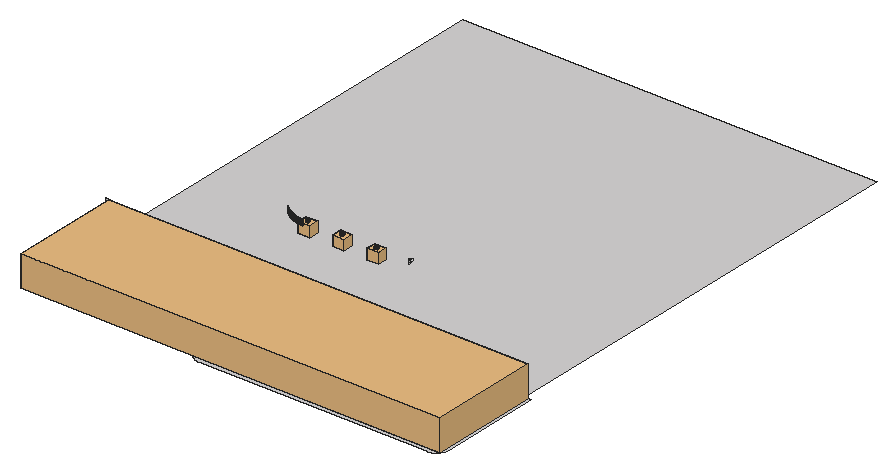
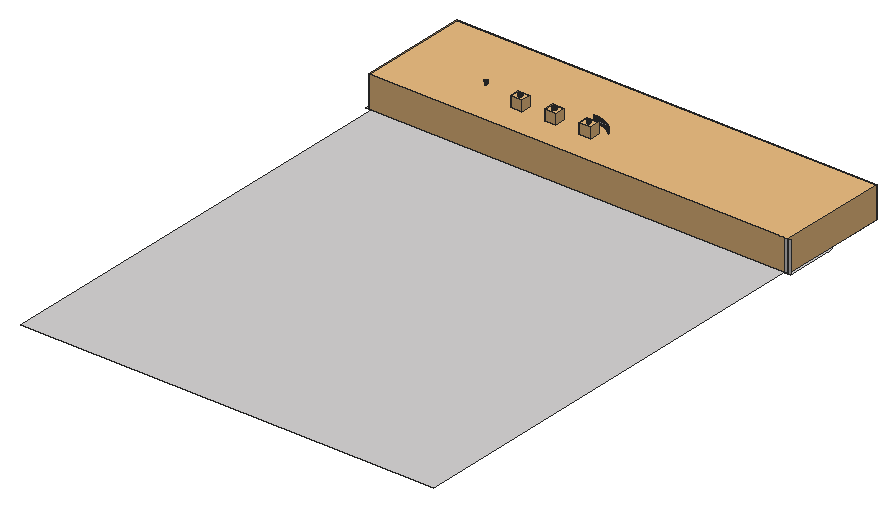
# SketchUp Ruby script. Lengths in inches.
U = 1.inch
M = Sketchup.active_model
def pt(a) = Geom::Point3d.new(a.map { |v| v * U })
def face(e, loops, mat)
  f = e.add_face(loops[0].map { |a| pt(a) })
  loops[1..].each { |l| e.add_face(l.map { |a| pt(a) }).erase! }
  f.material = f.back_material = mat if mat
  f
end
# faces: each face lists its corners as indices into pts; further lists are holes
def faces(e, pts, list, mat = nil) = list.each { |f| face(e, (f[0].is_a?(Array) ? f : [f]).map { |l| l.map { |i| pts[i] } }, mat) }
# xy, xz, yz: faces in a plane at the given z, y or x. An outline is a flat list of corners, or four numbers for a rectangle; further outlines are holes
def ring(l) = l.size == 4 ? [[l[0], l[1]], [l[2], l[1]], [l[2], l[3]], [l[0], l[3]]] : l.each_slice(2).to_a
def flat(e, list, mat, &to3) = list.each { |f| face(e, (f[0].is_a?(Array) ? f : [f]).map { |l| ring(l).map { |u, v| to3.(u, v) } }, mat) }
def xy(e, z, list, mat = nil) = flat(e, list, mat) { |x, y| [x, y, z] }
def xz(e, y, list, mat = nil) = flat(e, list, mat) { |x, z| [x, y, z] }
def yz(e, x, list, mat = nil) = flat(e, list, mat) { |y, z| [x, y, z] }
def lines(e, pts, list) = list.each { |a, b| e.add_line(pt(pts[a]), pt(pts[b])) }
# prism: a flat outline (further loops are holes) pulled along v
def prism(e, loops, v, mat = nil)
  f = face(e, loops, mat); d = Geom::Vector3d.new(v.map { |x| x * U })
  f.pushpull(f.normal.samedirection?(d) ? d.length : -d.length)
end
def box(e, o, s, mat = nil) = prism(e, [[o, [o[0] + s[0], o[1], o[2]], [o[0] + s[0], o[1] + s[1], o[2]], [o[0], o[1] + s[1], o[2]]]], [0, 0, s[2]], mat)
def at(x, y, z, deg = 0) = Geom::Transformation.translation(pt([x, y, z])) * Geom::Transformation.rotation(ORIGIN, Z_AXIS, deg.degrees)
def axes(o, x, y, z) = Geom::Transformation.new([*x, 0, *y, 0, *z, 0, *pt(o).to_a, 1])
def part(name) = M.definitions.add(name)
# library, detail: a bought-in or finely detailed component or shape, given as its bounding box
def library(name, o, s) = part(name).tap { |d| box(d.entities, o, s) }
def detail(e, o, s) = box(e.add_group.entities, o, s)
def put(e, d, t, mat = nil) = e.add_instance(d, t).tap { |i| i.material = mat if mat }
def group(e, t, mat = nil) = e.add_group.tap { |g| g.transformation = t; g.material = mat if mat }.entities
root = M.entities
M.materials.add("T METAL").color = [42, 41, 39]
M.materials.add("[Quartz Light Brown]").color = [215, 212, 212]
c1 = library("3",[-5.26,-4.28,-11.86],[13.52,11.56,11.86])
c2 = library("Group\#48",[0,0,0],[483,127.5,40])
xy(root,396,[[215.8,143,480.2,143,480.39,143.01,480.59,143.01,480.79,143.02,480.98,143.03,481.18,143.05,481.37,143.0625,481.57,143.08,481.76,143.1,481.96,143.13,482.15,143.16,482.35,143.18,482.54,143.22,482.73,143.25,482.93,143.29,483.5,143.41,483.88,143.51,484.07,143.5625,484.26,143.62,484.45,143.67,484.64,143.73,484.82,143.8,485.01,143.86,485.19,143.93,485.56,144.07,485.74,144.14,486.46,144.46,486.63,144.55,486.81,144.63,486.98,144.73,487.16,144.82,487.33,144.91,487.84,145.21,488,145.3125,488.17,145.42,488.33,145.53,488.5,145.64,488.82,145.86,488.97,145.98,489.29,146.22,489.44,146.34,489.59,146.47,489.74,146.59,490.04,146.85,490.18,146.99,490.33,147.12,490.47,147.26,490.61,147.39,490.74,147.53,490.88,147.67,491.01,147.82,491.15,147.96,491.41,148.26,491.53,148.41,491.66,148.56,491.78,148.71,492.02,149.03,492.14,149.18,492.36,149.5,492.47,149.67,492.58,149.83,492.6875,150,492.79,150.16,493.09,150.67,493.18,150.84,493.27,151.02,493.37,151.19,493.45,151.37,493.54,151.54,493.86,152.26,493.93,152.44,494.07,152.81,494.14,152.99,494.2,153.18,494.27,153.36,494.33,153.55,494.38,153.74,494.4375,153.93,494.49,154.12,494.59,154.5,494.71,155.07,494.75,155.27,494.78,155.46,494.82,155.65,494.84,155.85,494.87,156.04,494.9,156.24,494.92,156.43,494.9375,156.63,494.95,156.82,494.97,157.02,494.98,157.21,494.99,157.41,494.99,157.61,495,157.8,495,276.5,488,276.5,488,787,7,787,7,276.5,0,276.5,0,222.76,0.01,222.53,0.01,222.29,0.02,222.06,0.04,221.82,0.06,221.59,0.08,221.35,0.1,221.12,0.125,220.88,0.15,220.65,0.1875,220.42,0.22,220.18,0.3,219.72,0.35,219.49,0.39,219.26,0.44,219.03,0.5,218.8,0.55,218.57,0.61,218.34,0.68,218.11,0.74,217.89,0.81,217.66,0.88,217.4375,0.96,217.21,1.03,216.99,1.11,216.77,1.2,216.55,1.28,216.33,1.46,215.89,1.56,215.68,1.65,215.46,1.75,215.25,1.86,215.04,1.96,214.83,2.18,214.41,2.3,214.2,2.41,214,2.65,213.6,2.78,213.39,2.9,213.2,3.03,213,3.17,212.8,3.3,212.61,3.4375,212.42,3.58,212.23,3.72,212.04,3.86,211.86,4.01,211.67,4.16,211.49,4.3125,211.31,4.47,211.13,4.625,210.96,4.78,210.78,4.94,210.61,5.11,210.44,5.27,210.27,5.44,210.11,5.61,209.94,5.78,209.78,5.96,209.625,6.13,209.47,6.31,209.3125,6.49,209.16,6.67,209.01,6.86,208.86,7.04,208.72,7.23,208.58,7.42,208.4375,7.61,208.3,7.8,208.17,8,208.03,8.2,207.9,8.39,207.78,8.6,207.65,9,207.41,9.2,207.3,9.41,207.18,9.83,206.96,10.04,206.86,10.25,206.75,10.46,206.65,10.68,206.56,10.89,206.46,11.33,206.28,11.55,206.2,11.77,206.11,11.99,206.03,12.21,205.96,12.4375,205.88,12.66,205.81,12.89,205.74,13.11,205.68,13.34,205.61,13.57,205.55,13.8,205.5,14.03,205.44,14.26,205.39,14.49,205.35,14.72,205.3,15.18,205.22,15.42,205.1875,15.65,205.15,15.88,205.125,16.12,205.1,16.35,205.08,16.59,205.06,16.82,205.04,17.06,205.02,17.29,205.01,17.53,205.01,17.76,205,201,205,201,157.8,201.01,157.61,201.01,157.41,201.02,157.21,201.03,157.02,201.05,156.82,201.0625,156.63,201.08,156.43,201.1,156.24,201.13,156.04,201.16,155.85,201.18,155.65,201.22,155.46,201.25,155.27,201.29,155.07,201.41,154.5,201.51,154.12,201.5625,153.93,201.62,153.74,201.67,153.55,201.73,153.36,201.8,153.18,201.86,152.99,201.93,152.81,202.07,152.44,202.14,152.26,202.46,151.54,202.55,151.37,202.63,151.19,202.73,151.02,202.82,150.84,202.91,150.67,203.21,150.16,203.3125,150,203.42,149.83,203.53,149.67,203.64,149.5,203.86,149.18,203.98,149.03,204.22,148.71,204.34,148.56,204.47,148.41,204.59,148.26,204.85,147.96,204.99,147.82,205.12,147.67,205.26,147.53,205.39,147.39,205.53,147.26,205.67,147.12,205.82,146.99,205.96,146.85,206.26,146.59,206.41,146.47,206.56,146.34,206.71,146.22,207.03,145.98,207.18,145.86,207.5,145.64,207.67,145.53,207.83,145.42,208,145.3125,208.16,145.21,208.67,144.91,208.84,144.82,209.02,144.73,209.19,144.63,209.37,144.55,209.54,144.46,210.26,144.14,210.44,144.07,210.81,143.93,210.99,143.86,211.18,143.8,211.36,143.73,211.55,143.67,211.74,143.62,211.93,143.5625,212.12,143.51,212.5,143.41,213.07,143.29,213.27,143.25,213.46,143.22,213.65,143.18,213.85,143.16,214.04,143.13,214.24,143.1,214.43,143.08,214.63,143.0625,214.82,143.05,215.02,143.03,215.21,143.02,215.41,143.01,215.61,143.01]],"[Quartz Light Brown]")
xy(root,483,[[224.9375,287.7,224.78,287.71,224.47,287.77,224.32,287.82,224.18,287.88,224.04,287.95,223.9,288.03,223.77,288.12,223.65,288.22,223.54,288.33,223.44,288.45,223.26,288.71,223.19,288.85,223.13,288.99,223.08,289.14,223.04,289.29,223,289.61,223,289.76,223.01,289.92,223.04,290.08,223.07,290.23,223.12,290.38,223.18,290.52,223.25,290.66,223.33,290.8,223.42,290.93,223.52,291.05,223.63,291.16,223.75,291.26,223.875,291.35,224.01,291.4375,224.15,291.51,224.29,291.57,224.44,291.62,224.59,291.66,224.75,291.69,224.91,291.7,225.0625,291.7,225.22,291.6875,225.375,291.67,225.53,291.63,225.68,291.58,225.82,291.52,225.96,291.45,226.1,291.37,226.23,291.28,226.35,291.18,226.46,291.07,226.56,290.95,226.65,290.83,226.74,290.69,226.81,290.55,226.87,290.41,226.92,290.26,226.96,290.11,226.98,289.95,227,289.8,227,289.64,226.99,289.48,226.96,289.33,226.93,289.17,226.88,289.02,226.82,288.88,226.75,288.74,226.67,288.6,226.58,288.48,226.48,288.36,226.37,288.24,226.25,288.14,226.125,288.05,225.99,287.96,225.85,287.89,225.71,287.83,225.56,287.78,225.41,287.74,225.09,287.7],[264.77,287.7,264.61,287.71,264.31,287.77,264.16,287.82,264.01,287.88,263.87,287.95,263.74,288.03,263.61,288.12,263.49,288.22,263.375,288.33,263.27,288.45,263.18,288.58,263.1,288.71,263.02,288.85,262.96,288.99,262.91,289.14,262.875,289.29,262.85,289.45,262.84,289.61,262.83,289.76,262.87,290.08,262.9,290.23,262.95,290.38,263.01,290.52,263.08,290.66,263.16,290.8,263.25,290.93,263.35,291.05,263.46,291.16,263.58,291.26,263.71,291.35,263.84,291.4375,263.98,291.51,264.125,291.57,264.27,291.62,264.43,291.66,264.58,291.69,264.74,291.7,264.9,291.7,265.05,291.6875,265.21,291.67,265.36,291.63,265.51,291.58,265.66,291.52,265.8,291.45,265.93,291.37,266.06,291.28,266.18,291.18,266.29,291.07,266.49,290.83,266.57,290.69,266.64,290.55,266.7,290.41,266.75,290.26,266.79,290.11,266.82,289.95,266.83,289.8,266.83,289.64,266.82,289.48,266.8,289.33,266.76,289.17,266.72,289.02,266.66,288.88,266.59,288.74,266.51,288.6,266.41,288.48,266.3125,288.36,266.2,288.24,266.08,288.14,265.96,288.05,265.82,287.96,265.69,287.89,265.54,287.83,265.39,287.78,265.24,287.74,265.08,287.72,264.93,287.7],[304.6,287.7,304.45,287.71,304.29,287.74,304.14,287.77,303.99,287.82,303.84,287.88,303.7,287.95,303.57,288.03,303.44,288.12,303.32,288.22,303.21,288.33,303.11,288.45,303.01,288.58,302.93,288.71,302.86,288.85,302.8,288.99,302.75,289.14,302.71,289.29,302.68,289.45,302.67,289.61,302.67,289.76,302.68,289.92,302.7,290.08,302.78,290.38,302.84,290.52,302.91,290.66,302.99,290.8,303.09,290.93,303.1875,291.05,303.3,291.16,303.42,291.26,303.54,291.35,303.68,291.4375,303.81,291.51,303.96,291.57,304.11,291.62,304.26,291.66,304.42,291.69,304.57,291.7,304.73,291.7,304.89,291.6875,305.04,291.67,305.19,291.63,305.34,291.58,305.49,291.52,305.63,291.45,305.76,291.37,305.89,291.28,306.01,291.18,306.125,291.07,306.23,290.95,306.32,290.83,306.48,290.55,306.54,290.41,306.59,290.26,306.625,290.11,306.65,289.95,306.66,289.8,306.67,289.64,306.65,289.48,306.63,289.33,306.6,289.17,306.55,289.02,306.49,288.88,306.42,288.74,306.34,288.6,306.25,288.48,306.15,288.36,306.04,288.24,305.92,288.14,305.66,287.96,305.52,287.89,305.375,287.83,305.23,287.78,305.07,287.74,304.92,287.72,304.76,287.7],[344.4375,287.7,344.28,287.71,343.97,287.77,343.82,287.82,343.68,287.88,343.54,287.95,343.4,288.03,343.27,288.12,343.15,288.22,343.04,288.33,342.94,288.45,342.76,288.71,342.69,288.85,342.63,288.99,342.58,289.14,342.54,289.29,342.5,289.61,342.5,289.76,342.51,289.92,342.54,290.08,342.57,290.23,342.62,290.38,342.68,290.52,342.75,290.66,342.83,290.8,342.92,290.93,343.02,291.05,343.13,291.16,343.25,291.26,343.375,291.35,343.51,291.4375,343.65,291.51,343.79,291.57,343.94,291.62,344.09,291.66,344.25,291.69,344.41,291.7,344.5625,291.7,344.72,291.6875,344.875,291.67,345.03,291.63,345.18,291.58,345.32,291.52,345.46,291.45,345.6,291.37,345.73,291.28,345.85,291.18,345.96,291.07,346.06,290.95,346.15,290.83,346.24,290.69,346.31,290.55,346.37,290.41,346.42,290.26,346.46,290.11,346.48,289.95,346.5,289.8,346.5,289.64,346.49,289.48,346.46,289.33,346.43,289.17,346.38,289.02,346.32,288.88,346.25,288.74,346.17,288.6,346.08,288.48,345.98,288.36,345.87,288.24,345.75,288.14,345.625,288.05,345.49,287.96,345.35,287.89,345.21,287.83,345.06,287.78,344.91,287.74,344.59,287.7]],"[Quartz Light Brown]")
xz(root,276.5,[[0,396,7,432]],"[Quartz Light Brown]")
xz(root,282.7,[[224.5,480,225,486]],"[Quartz Light Brown]")
xz(root,287.7,[[224.9375,480,225.09,483],[264.77,480,264.93,483],[304.6,480,304.76,483]],"[Quartz Light Brown]")
xz(root,291.7,[[224.91,480,225.0625,483],[264.74,480,264.9,483],[304.57,480,304.73,483],[344.41,480,344.5625,483]],"[Quartz Light Brown]")
yz(root,223,[[289.61,480,289.76,483]],"[Quartz Light Brown]")
yz(root,227,[[289.64,480,289.8,483]],"[Quartz Light Brown]")
yz(root,266.83,[[289.64,480,289.8,483]],"[Quartz Light Brown]")
yz(root,302.67,[[289.61,480,289.76,483]],"[Quartz Light Brown]")
yz(root,342.5,[[289.61,480,289.76,483]],"[Quartz Light Brown]")
p = [[223.01,282.75,480],[223.51,282.73,480],[223.51,282.73,486],[223.01,282.75,486],[224.01,282.71,480],[224.01,282.71,486],
  [224.5,282.7,480],[224.5,282.7,486],[221.52,282.86,480],[222.02,282.82,480],[222.02,282.82,486],[221.52,282.86,486],
  [222.51,282.78,480],[222.51,282.78,486],[220.53,282.96,480],[221.03,282.91,480],[221.03,282.91,486],[220.53,282.96,486],
  [219.55,283.09,480],[220.04,283.03,480],[220.04,283.03,486],[219.55,283.09,486],[219.06,283.17,480],[219.06,283.17,486],
  [218.08,283.34,480],[218.56,283.25,480],[218.56,283.25,486],[218.08,283.34,486],[217.59,283.43,480],[217.59,283.43,486],
  [217.1,283.53,480],[217.1,283.53,486],[216.61,283.64,480],[216.61,283.64,486],[216.13,283.75,480],[216.13,283.75,486],
  [215.65,283.87,480],[215.65,283.87,486],[215.16,284,480],[215.16,284,486],[214.69,284.13,480],[214.69,284.13,486],
  [214.21,284.27,480],[214.21,284.27,486],[213.73,284.41,480],[213.73,284.41,486],[213.26,284.5625,480],[213.26,284.5625,486],
  [212.79,284.72,480],[212.79,284.72,486],[212.32,284.88,480],[212.32,284.88,486],[211.85,285.05,480],[211.85,285.05,486],
  [211.38,285.22,480],[211.38,285.22,486],[210.92,285.41,480],[210.92,285.41,486],[210.46,285.59,480],[210.46,285.59,486],
  [210,285.79,480],[210,285.79,486],[209.54,285.99,480],[209.54,285.99,486],[209.09,286.19,480],[209.09,286.19,486],
  [208.64,286.4,480],[208.64,286.4,486],[208.19,286.62,480],[208.19,286.62,486],[207.75,286.84,480],[207.75,286.84,486],
  [207.31,287.07,480],[207.31,287.07,486],[206.87,287.31,480],[206.87,287.31,486],[206.43,287.55,480],[206.43,287.55,486],
  [206,287.79,480],[206,287.79,486],[224.625,287.74,480],[224.47,287.77,480],[224.47,287.77,483],[224.625,287.74,483],
  [224.78,287.71,480],[224.78,287.71,483],[224.9375,287.7,480],[224.9375,287.7,483],[225.25,287.72,480],[225.09,287.7,480],
  [225.09,287.7,483],[225.25,287.72,483],[225.41,287.74,480],[225.41,287.74,483],[225.56,287.78,480],[225.56,287.78,483],
  [264.46,287.74,480],[264.31,287.77,480],[264.31,287.77,483],[264.46,287.74,483],[264.61,287.71,480],[264.61,287.71,483],
  [264.77,287.7,480],[264.77,287.7,483],[265.08,287.72,480],[264.93,287.7,480],[264.93,287.7,483],[265.08,287.72,483],
  [265.24,287.74,480],[265.24,287.74,483],[265.39,287.78,480],[265.39,287.78,483],[304.29,287.74,480],[304.14,287.77,480],
  [304.14,287.77,483],[304.29,287.74,483],[304.45,287.71,480],[304.45,287.71,483],[304.6,287.7,480],[304.6,287.7,483],
  [304.92,287.72,480],[304.76,287.7,480],[304.76,287.7,483],[304.92,287.72,483],[305.07,287.74,480],[305.07,287.74,483],
  [305.23,287.78,480],[305.23,287.78,483],[344.125,287.74,480],[343.97,287.77,480],[343.97,287.77,483],[344.125,287.74,483],
  [344.28,287.71,480],[344.28,287.71,483],[344.4375,287.7,480],[344.4375,287.7,483],[205.57,288.04,480],[205.57,288.04,486],
  [224.32,287.82,480],[224.18,287.88,480],[224.18,287.88,483],[224.32,287.82,483],[225.71,287.83,480],[225.71,287.83,483],
  [225.85,287.89,480],[225.85,287.89,483],[264.16,287.82,480],[264.01,287.88,480],[264.01,287.88,483],[264.16,287.82,483],
  [265.54,287.83,480],[265.54,287.83,483],[265.69,287.89,480],[265.69,287.89,483],[303.99,287.82,480],[303.84,287.88,480],
  [303.84,287.88,483],[303.99,287.82,483],[305.375,287.83,480],[305.375,287.83,483],[305.52,287.89,480],[305.52,287.89,483],
  [343.82,287.82,480],[343.68,287.88,480],[343.68,287.88,483],[343.82,287.82,483],[224.04,287.95,480],[223.9,288.03,480],
  [223.9,288.03,483],[224.04,287.95,483],[225.99,287.96,480],[225.99,287.96,483],[263.87,287.95,480],[263.74,288.03,480],
  [263.74,288.03,483],[263.87,287.95,483],[265.82,287.96,480],[265.82,287.96,483],[303.7,287.95,480],[303.57,288.03,480],
  [303.57,288.03,483],[303.7,287.95,483],[305.66,287.96,480],[305.66,287.96,483],[343.54,287.95,480],[343.4,288.03,480],
  [343.4,288.03,483],[343.54,287.95,483],[205.15,288.3,480],[205.15,288.3,486],[223.77,288.12,480],[223.77,288.12,483],
  [226.125,288.05,480],[226.125,288.05,483],[226.25,288.14,480],[226.25,288.14,483],[263.61,288.12,480],[263.61,288.12,483],
  [265.96,288.05,480],[265.96,288.05,483],[266.08,288.14,480],[266.08,288.14,483],[303.44,288.12,480],[303.44,288.12,483],
  [305.79,288.05,480],[305.79,288.05,483],[305.92,288.14,480],[305.92,288.14,483],[343.27,288.12,480],[343.27,288.12,483],
  [223.65,288.22,480],[223.65,288.22,483],[226.37,288.24,480],[226.37,288.24,483],[263.49,288.22,480],[263.49,288.22,483],
  [266.2,288.24,480],[266.2,288.24,483],[303.32,288.22,480],[303.32,288.22,483],[306.04,288.24,480],[306.04,288.24,483],
  [343.15,288.22,480],[343.15,288.22,483],[223.54,288.33,480],[223.54,288.33,483],[226.48,288.36,480],[226.48,288.36,483],
  [263.375,288.33,480],[263.375,288.33,483],[266.3125,288.36,480],[266.3125,288.36,483],[303.21,288.33,480],[303.21,288.33,483],
  [306.15,288.36,480],[306.15,288.36,483],[343.04,288.33,480],[343.04,288.33,483],[204.72,288.5625,480],[204.72,288.5625,486],
  [223.44,288.45,480],[223.44,288.45,483],[263.27,288.45,480],[263.27,288.45,483],[303.11,288.45,480],[303.11,288.45,483],
  [342.94,288.45,480],[342.94,288.45,483],[226.58,288.48,480],[226.58,288.48,483],[266.41,288.48,480],[266.41,288.48,483],
  [306.25,288.48,480],[306.25,288.48,483],[223.35,288.58,480],[223.35,288.58,483],[226.67,288.6,480],[226.67,288.6,483],
  [263.18,288.58,480],[263.18,288.58,483],[266.51,288.6,480],[266.51,288.6,483],[303.01,288.58,480],[303.01,288.58,483],
  [306.34,288.6,480],[306.34,288.6,483],[342.85,288.58,480],[342.85,288.58,483],[204.3,288.83,480],[204.3,288.83,486],
  [223.26,288.71,480],[223.26,288.71,483],[226.75,288.74,480],[226.75,288.74,483],[263.1,288.71,480],[263.1,288.71,483],
  [266.59,288.74,480],[266.59,288.74,483],[302.93,288.71,480],[302.93,288.71,483],[306.42,288.74,480],[306.42,288.74,483],
  [342.76,288.71,480],[342.76,288.71,483],[223.19,288.85,480],[223.19,288.85,483],[226.82,288.88,480],[226.82,288.88,483],
  [263.02,288.85,480],[263.02,288.85,483],[266.66,288.88,480],[266.66,288.88,483],[302.86,288.85,480],[302.86,288.85,483],
  [306.49,288.88,480],[306.49,288.88,483],[342.69,288.85,480],[342.69,288.85,483],[203.89,289.11,480],[203.89,289.11,486],
  [223.13,288.99,480],[223.13,288.99,483],[262.96,288.99,480],[262.96,288.99,483],[302.8,288.99,480],[302.8,288.99,483],
  [342.63,288.99,480],[342.63,288.99,483],[226.88,289.02,480],[226.88,289.02,483],[266.72,289.02,480],[266.72,289.02,483],
  [306.55,289.02,480],[306.55,289.02,483],[223.08,289.14,480],[223.08,289.14,483],[226.93,289.17,480],[226.93,289.17,483],
  [262.91,289.14,480],[262.91,289.14,483],[266.76,289.17,480],[266.76,289.17,483],[302.75,289.14,480],[302.75,289.14,483],
  [306.6,289.17,480],[306.6,289.17,483],[342.58,289.14,480],[342.58,289.14,483],[203.48,289.38,480],[203.48,289.38,486],
  [223.04,289.29,480],[223.04,289.29,483],[262.875,289.29,480],[262.875,289.29,483],[302.71,289.29,480],[302.71,289.29,483],
  [342.54,289.29,480],[342.54,289.29,483],[226.96,289.33,480],[226.96,289.33,483],[266.8,289.33,480],[266.8,289.33,483],
  [306.63,289.33,480],[306.63,289.33,483],[223.02,289.45,480],[223.02,289.45,483],[226.99,289.48,480],[226.99,289.48,483],
  [262.85,289.45,480],[262.85,289.45,483],[266.82,289.48,480],[266.82,289.48,483],[302.68,289.45,480],[302.68,289.45,483],
  [306.65,289.48,480],[306.65,289.48,483],[342.52,289.45,480],[342.52,289.45,483],[203.07,289.67,480],[203.07,289.67,486],
  [223,289.61,480],[223,289.61,483],[262.84,289.61,480],[262.84,289.61,483],[302.67,289.61,480],[302.67,289.61,483],
  [342.5,289.61,480],[342.5,289.61,483],[227,289.64,480],[227,289.64,483],[266.83,289.64,480],[266.83,289.64,483],
  [306.67,289.64,480],[306.67,289.64,483],[262.83,289.76,480],[262.83,289.76,483],[306.66,289.8,480],[306.66,289.8,483],
  [202.66,289.96,480],[202.66,289.96,486],[223,289.76,480],[223.01,289.92,480],[223.01,289.92,483],[223,289.76,483],
  [226.98,289.95,480],[227,289.8,480],[227,289.8,483],[226.98,289.95,483],[262.85,289.92,480],[262.85,289.92,483],
  [266.82,289.95,480],[266.83,289.8,480],[266.83,289.8,483],[266.82,289.95,483],[302.67,289.76,480],[302.68,289.92,480],
  [302.68,289.92,483],[302.67,289.76,483],[306.65,289.95,480],[306.65,289.95,483],[342.5,289.76,480],[342.51,289.92,480],
  [342.51,289.92,483],[342.5,289.76,483],[223.04,290.08,480],[223.04,290.08,483],[262.87,290.08,480],[262.87,290.08,483],
  [302.7,290.08,480],[302.7,290.08,483],[342.54,290.08,480],[342.54,290.08,483],[202.26,290.25,480],[202.26,290.25,486],
  [226.96,290.11,480],[226.96,290.11,483],[266.79,290.11,480],[266.79,290.11,483],[306.625,290.11,480],[306.625,290.11,483],
  [223.07,290.23,480],[223.07,290.23,483],[226.92,290.26,480],[226.92,290.26,483],[262.9,290.23,480],[262.9,290.23,483],
  [266.75,290.26,480],[266.75,290.26,483],[302.74,290.23,480],[302.74,290.23,483],[306.59,290.26,480],[306.59,290.26,483],
  [342.57,290.23,480],[342.57,290.23,483],[223.12,290.38,480],[223.12,290.38,483],[262.95,290.38,480],[262.95,290.38,483],
  [302.78,290.38,480],[302.78,290.38,483],[342.62,290.38,480],[342.62,290.38,483],[201.87,290.55,480],[201.87,290.55,486],
  [226.87,290.41,480],[226.87,290.41,483],[266.7,290.41,480],[266.7,290.41,483],[306.54,290.41,480],[306.54,290.41,483],
  [223.18,290.52,480],[223.18,290.52,483],[226.81,290.55,480],[226.81,290.55,483],[263.01,290.52,480],[263.01,290.52,483],
  [266.64,290.55,480],[266.64,290.55,483],[302.84,290.52,480],[302.84,290.52,483],[306.48,290.55,480],[306.48,290.55,483],
  [342.68,290.52,480],[342.68,290.52,483],[223.25,290.66,480],[223.25,290.66,483],[263.08,290.66,480],[263.08,290.66,483],
  [302.91,290.66,480],[302.91,290.66,483],[342.75,290.66,480],[342.75,290.66,483],[201.47,290.86,480],[201.47,290.86,486],
  [226.74,290.69,480],[226.74,290.69,483],[266.57,290.69,480],[266.57,290.69,483],[306.4,290.69,480],[306.4,290.69,483],
  [223.33,290.8,480],[223.33,290.8,483],[226.65,290.83,480],[226.65,290.83,483],[263.16,290.8,480],[263.16,290.8,483],
  [266.49,290.83,480],[266.49,290.83,483],[302.99,290.8,480],[302.99,290.8,483],[306.32,290.83,480],[306.32,290.83,483],
  [342.83,290.8,480],[342.83,290.8,483],[223.42,290.93,480],[223.42,290.93,483],[226.56,290.95,480],[226.56,290.95,483],
  [263.25,290.93,480],[263.25,290.93,483],[266.39,290.95,480],[266.39,290.95,483],[303.09,290.93,480],[303.09,290.93,483],
  [306.23,290.95,480],[306.23,290.95,483],[342.92,290.93,480],[342.92,290.93,483],[201.09,291.17,480],[201.09,291.17,486],
  [223.52,291.05,480],[223.52,291.05,483],[263.35,291.05,480],[263.35,291.05,483],[303.1875,291.05,480],[303.1875,291.05,483],
  [343.02,291.05,480],[343.02,291.05,483],[223.63,291.16,480],[223.63,291.16,483],[226.46,291.07,480],[226.46,291.07,483],
  [263.46,291.16,480],[263.46,291.16,483],[266.29,291.07,480],[266.29,291.07,483],[303.3,291.16,480],[303.3,291.16,483],
  [306.125,291.07,480],[306.125,291.07,483],[343.13,291.16,480],[343.13,291.16,483],[226.35,291.18,480],[226.35,291.18,483],
  [266.18,291.18,480],[266.18,291.18,483],[306.01,291.18,480],[306.01,291.18,483],[200.7,291.49,480],[200.7,291.49,486],
  [223.75,291.26,480],[223.75,291.26,483],[226.23,291.28,480],[226.23,291.28,483],[263.58,291.26,480],[263.58,291.26,483],
  [266.06,291.28,480],[266.06,291.28,483],[303.42,291.26,480],[303.42,291.26,483],[305.89,291.28,480],[305.89,291.28,483],
  [343.25,291.26,480],[343.25,291.26,483],[223.875,291.35,480],[223.875,291.35,483],[226.1,291.37,480],[226.1,291.37,483],
  [263.71,291.35,480],[263.71,291.35,483],[265.93,291.37,480],[265.93,291.37,483],[303.54,291.35,480],[303.54,291.35,483],
  [305.76,291.37,480],[305.76,291.37,483],[343.375,291.35,480],[343.375,291.35,483],[224.01,291.4375,480],[224.01,291.4375,483],
  [224.15,291.51,480],[224.15,291.51,483],[225.96,291.45,480],[225.96,291.45,483],[263.84,291.4375,480],[263.84,291.4375,483],
  [263.98,291.51,480],[263.98,291.51,483],[265.8,291.45,480],[265.8,291.45,483],[303.68,291.4375,480],[303.68,291.4375,483],
  [303.81,291.51,480],[303.81,291.51,483],[305.63,291.45,480],[305.63,291.45,483],[343.51,291.4375,480],[343.51,291.4375,483],
  [343.65,291.51,480],[343.65,291.51,483],[200.32,291.81,480],[200.32,291.81,486],[224.29,291.57,480],[224.29,291.57,483],
  [225.68,291.58,480],[225.82,291.52,480],[225.82,291.52,483],[225.68,291.58,483],[264.125,291.57,480],[264.125,291.57,483],
  [265.51,291.58,480],[265.66,291.52,480],[265.66,291.52,483],[265.51,291.58,483],[303.96,291.57,480],[303.96,291.57,483],
  [305.34,291.58,480],[305.49,291.52,480],[305.49,291.52,483],[305.34,291.58,483],[343.79,291.57,480],[343.79,291.57,483],
  [224.44,291.62,480],[224.44,291.62,483],[224.59,291.66,480],[224.59,291.66,483],[225.375,291.67,480],[225.53,291.63,480],
  [225.53,291.63,483],[225.375,291.67,483],[264.27,291.62,480],[264.27,291.62,483],[264.43,291.66,480],[264.43,291.66,483],
  [265.21,291.67,480],[265.36,291.63,480],[265.36,291.63,483],[265.21,291.67,483],[304.11,291.62,480],[304.11,291.62,483],
  [304.26,291.66,480],[304.26,291.66,483],[305.04,291.67,480],[305.19,291.63,480],[305.19,291.63,483],[305.04,291.67,483],
  [343.94,291.62,480],[343.94,291.62,483],[344.09,291.66,480],[344.09,291.66,483],[224.75,291.69,480],[224.75,291.69,483],
  [224.91,291.7,480],[224.91,291.7,483],[225.0625,291.7,480],[225.22,291.6875,480],[225.22,291.6875,483],[225.0625,291.7,483],
  [264.58,291.69,480],[264.58,291.69,483],[264.74,291.7,480],[264.74,291.7,483],[264.9,291.7,480],[265.05,291.6875,480],
  [265.05,291.6875,483],[264.9,291.7,483],[304.42,291.69,480],[304.42,291.69,483],[304.57,291.7,480],[304.57,291.7,483],
  [304.73,291.7,480],[304.89,291.6875,480],[304.89,291.6875,483],[304.73,291.7,483],[344.25,291.69,480],[344.25,291.69,483],
  [344.41,291.7,480],[344.41,291.7,483],[199.94,292.13,480],[199.94,292.13,486],[199.57,292.46,480],[199.57,292.46,486],
  [199.21,292.8,480],[199.21,292.8,486],[198.84,293.14,480],[198.84,293.14,486],[198.48,293.48,480],[198.48,293.48,486]]
faces(root,p,[[0,1,2,3],[1,4,5,2],[4,6,7,5],[8,9,10,11],[9,12,13,10],[12,0,3,13],[14,15,16,17],[15,8,11,16],
  [18,19,20,21],[19,14,17,20],[22,18,21,23],[24,25,26,27],[25,22,23,26],[28,24,27,29],[30,28,29,31],[32,30,31,33],
  [34,32,33,35],[36,34,35,37],[38,36,37,39],[40,38,39,41],[42,40,41,43],[44,42,43,45],[46,44,45,47],[48,46,47,49],
  [50,48,49,51],[52,50,51,53],[54,52,53,55],[56,54,55,57],[58,56,57,59],[60,58,59,61],[62,60,61,63],[64,62,63,65],
  [66,64,65,67],[68,66,67,69],[70,68,69,71],[72,70,71,73],[74,72,73,75],[76,74,75,77],[78,76,77,79],[80,81,82,83],
  [84,80,83,85],[86,84,85,87],[88,89,90,91],[92,88,91,93],[94,92,93,95],[96,97,98,99],[100,96,99,101],[102,100,101,103],
  [104,105,106,107],[108,104,107,109],[110,108,109,111],[112,113,114,115],[116,112,115,117],[118,116,117,119],[120,121,122,123],[124,120,123,125],
  [126,124,125,127],[128,129,130,131],[132,128,131,133],[134,132,133,135],[136,78,79,137],[138,139,140,141],[81,138,141,82],[142,94,95,143],
  [144,142,143,145],[146,147,148,149],[97,146,149,98],[150,110,111,151],[152,150,151,153],[154,155,156,157],[113,154,157,114],[158,126,127,159],
  [160,158,159,161],[162,163,164,165],[129,162,165,130],[166,167,168,169],[139,166,169,140],[170,144,145,171],[172,173,174,175],[147,172,175,148],
  [176,152,153,177],[178,179,180,181],[155,178,181,156],[182,160,161,183],[184,185,186,187],[163,184,187,164],[188,136,137,189],[167,190,191,168],
  [192,170,171,193],[194,192,193,195],[173,196,197,174],[198,176,177,199],[200,198,199,201],[179,202,203,180],[204,182,183,205],[206,204,205,207],
  [185,208,209,186],[190,210,211,191],[212,194,195,213],[196,214,215,197],[216,200,201,217],[202,218,219,203],[220,206,207,221],[208,222,223,209],
  [210,224,225,211],[226,212,213,227],[214,228,229,215],[230,216,217,231],[218,232,233,219],[234,220,221,235],[222,236,237,223],[238,188,189,239],
  [224,240,241,225],[228,242,243,229],[232,244,245,233],[236,246,247,237],[248,226,227,249],[250,230,231,251],[252,234,235,253],[240,254,255,241],
  [256,248,249,257],[242,258,259,243],[260,250,251,261],[244,262,263,245],[264,252,253,265],[246,266,267,247],[268,238,239,269],[254,270,271,255],
  [272,256,257,273],[258,274,275,259],[276,260,261,277],[262,278,279,263],[280,264,265,281],[266,282,283,267],[270,284,285,271],[286,272,273,287],
  [274,288,289,275],[290,276,277,291],[278,292,293,279],[294,280,281,295],[282,296,297,283],[298,268,269,299],[284,300,301,285],[288,302,303,289],
  [292,304,305,293],[296,306,307,297],[308,286,287,309],[310,290,291,311],[312,294,295,313],[300,314,315,301],[316,308,309,317],[302,318,319,303],
  [320,310,311,321],[304,322,323,305],[324,312,313,325],[306,326,327,307],[328,298,299,329],[314,330,331,315],[318,332,333,319],[322,334,335,323],
  [326,336,337,327],[338,316,317,339],[340,320,321,341],[342,324,325,343],[330,344,345,331],[346,338,339,347],[332,348,349,333],[350,340,341,351],
  [334,352,353,335],[354,342,343,355],[336,356,357,337],[358,328,329,359],[344,360,361,345],[348,362,363,349],[352,364,365,353],[356,366,367,357],
  [368,346,347,369],[370,350,351,371],[372,354,355,373],[362,374,375,363],[376,372,373,377],[378,358,359,379],[380,381,382,383],[384,385,386,387],
  [374,388,389,375],[390,391,392,393],[394,395,396,397],[398,376,377,399],[400,401,402,403],[381,404,405,382],[388,406,407,389],[395,408,409,396],
  [401,410,411,402],[412,378,379,413],[414,384,387,415],[416,390,393,417],[418,398,399,419],[404,420,421,405],[422,414,415,423],[406,424,425,407],
  [426,416,417,427],[408,428,429,409],[430,418,419,431],[410,432,433,411],[420,434,435,421],[424,436,437,425],[428,438,439,429],[432,440,441,433],
  [442,412,413,443],[444,422,423,445],[446,426,427,447],[448,430,431,449],[434,450,451,435],[452,444,445,453],[436,454,455,437],[456,446,447,457],
  [438,458,459,439],[460,448,449,461],[440,462,463,441],[450,464,465,451],[454,466,467,455],[458,468,469,459],[462,470,471,463],[472,442,443,473],
  [474,452,453,475],[476,456,457,477],[478,460,461,479],[464,480,481,465],[482,474,475,483],[466,484,485,467],[486,476,477,487],[468,488,489,469],
  [490,478,479,491],[470,492,493,471],[480,494,495,481],[496,482,483,497],[484,498,499,485],[500,486,487,501],[488,502,503,489],[504,490,491,505],
  [492,506,507,493],[508,472,473,509],[494,510,511,495],[498,512,513,499],[502,514,515,503],[506,516,517,507],[510,518,519,511],[520,496,497,521],
  [512,522,523,513],[524,500,501,525],[514,526,527,515],[528,504,505,529],[516,530,531,517],[532,520,521,533],[534,524,525,535],[536,528,529,537],
  [538,508,509,539],[518,540,541,519],[542,532,533,543],[522,544,545,523],[546,534,535,547],[526,548,549,527],[550,536,537,551],[530,552,553,531],
  [540,554,555,541],[556,542,543,557],[544,558,559,545],[560,546,547,561],[548,562,563,549],[564,550,551,565],[552,566,567,553],[554,568,569,555],
  [568,570,571,569],[572,556,557,573],[558,574,575,559],[574,576,577,575],[578,560,561,579],[562,580,581,563],[580,582,583,581],[584,564,565,585],
  [566,586,587,567],[586,588,589,587],[590,538,539,591],[570,592,593,571],[594,595,596,597],[595,572,573,596],[576,598,599,577],[600,601,602,603],
  [601,578,579,602],[582,604,605,583],[606,607,608,609],[607,584,585,608],[588,610,611,589],[592,612,613,593],[612,614,615,613],[616,617,618,619],
  [617,594,597,618],[598,620,621,599],[620,622,623,621],[624,625,626,627],[625,600,603,626],[604,628,629,605],[628,630,631,629],[632,633,634,635],
  [633,606,609,634],[610,636,637,611],[636,638,639,637],[614,640,641,615],[640,642,643,641],[644,645,646,647],[645,616,619,646],[622,648,649,623],
  [648,650,651,649],[652,653,654,655],[653,624,627,654],[630,656,657,631],[656,658,659,657],[660,661,662,663],[661,632,635,662],[638,664,665,639],
  [664,666,667,665],[668,590,591,669],[670,668,669,671],[672,670,671,673],[674,672,673,675],[676,674,675,677]],"[Quartz Light Brown]")
put(root,c1,at(223.5,288.2,481.25),"[Quartz Light Brown]")
put(root,c2,axes([3.57,148.36,396],[1.01002,0,0],[0,1.005,0],[0,0,0.9]),"T METAL")
put(root,c1,at(263.33,288.2,481.25),"[Quartz Light Brown]")
put(root,c1,at(303.17,288.2,481.25),"[Quartz Light Brown]")
